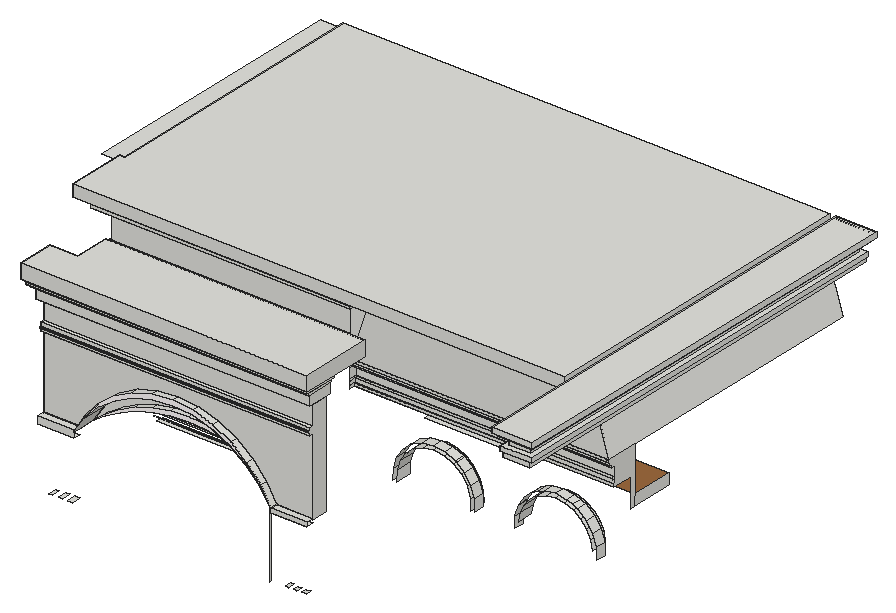
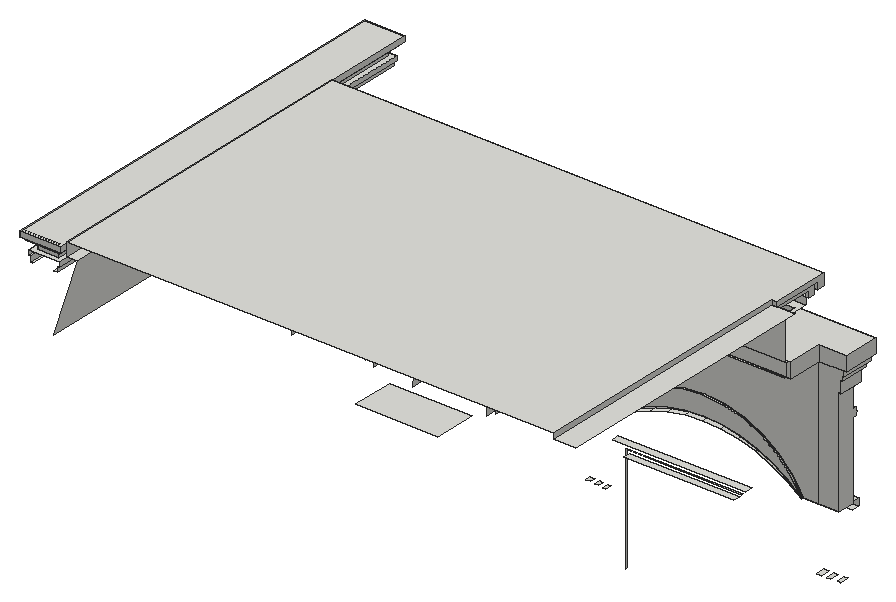
# SketchUp Ruby script. Lengths in millimetres.
U = 1.mm
M = Sketchup.active_model
def pt(a) = Geom::Point3d.new(a.map { |v| v * U })
def face(e, loops, mat)
  f = e.add_face(loops[0].map { |a| pt(a) })
  loops[1..].each { |l| e.add_face(l.map { |a| pt(a) }).erase! }
  f.material = f.back_material = mat if mat
  f
end
# faces: each face lists its corners as indices into pts; further lists are holes
def faces(e, pts, list, mat = nil) = list.each { |f| face(e, (f[0].is_a?(Array) ? f : [f]).map { |l| l.map { |i| pts[i] } }, mat) }
# xy, xz, yz: faces in a plane at the given z, y or x. An outline is a flat list of corners, or four numbers for a rectangle; further outlines are holes
def ring(l) = l.size == 4 ? [[l[0], l[1]], [l[2], l[1]], [l[2], l[3]], [l[0], l[3]]] : l.each_slice(2).to_a
def flat(e, list, mat, &to3) = list.each { |f| face(e, (f[0].is_a?(Array) ? f : [f]).map { |l| ring(l).map { |u, v| to3.(u, v) } }, mat) }
def xy(e, z, list, mat = nil) = flat(e, list, mat) { |x, y| [x, y, z] }
def xz(e, y, list, mat = nil) = flat(e, list, mat) { |x, z| [x, y, z] }
def yz(e, x, list, mat = nil) = flat(e, list, mat) { |y, z| [x, y, z] }
def lines(e, pts, list) = list.each { |a, b| e.add_line(pt(pts[a]), pt(pts[b])) }
# prism: a flat outline (further loops are holes) pulled along v
def prism(e, loops, v, mat = nil)
  f = face(e, loops, mat); d = Geom::Vector3d.new(v.map { |x| x * U })
  f.pushpull(f.normal.samedirection?(d) ? d.length : -d.length)
end
def box(e, o, s, mat = nil) = prism(e, [[o, [o[0] + s[0], o[1], o[2]], [o[0] + s[0], o[1] + s[1], o[2]], [o[0], o[1] + s[1], o[2]]]], [0, 0, s[2]], mat)
def at(x, y, z, deg = 0) = Geom::Transformation.translation(pt([x, y, z])) * Geom::Transformation.rotation(ORIGIN, Z_AXIS, deg.degrees)
def axes(o, x, y, z) = Geom::Transformation.new([*x, 0, *y, 0, *z, 0, *pt(o).to_a, 1])
def part(name) = M.definitions.add(name)
# library, detail: a bought-in or finely detailed component or shape, given as its bounding box
def library(name, o, s) = part(name).tap { |d| box(d.entities, o, s) }
def detail(e, o, s) = box(e.add_group.entities, o, s)
def put(e, d, t, mat = nil) = e.add_instance(d, t).tap { |i| i.material = mat if mat }
def group(e, t, mat = nil) = e.add_group.tap { |g| g.transformation = t; g.material = mat if mat }.entities
root = M.entities
M.materials.add("[0010_Snow]").color = [255, 250, 250]
M.materials.add("[Wood Floor]").color = [155, 105, 61]
xy(root,6858,[[4330.2,9852.4,4415.9,10085.7],[4585.1,9852.4,4702.2,10104.8],[4850.6,9852.4,4980.7,10104.8],[10956.8,9852.4,11053.6,10033.3]])
xy(root,6861.6,[[11185.3,9852.4,11289.9,10007.9]])
xy(root,6872.3,[[11425.8,9852.4,11548,9993.6]])
xy(root,8639.6,[[4179.9,9646,5191.1,9852.4]])
xy(root,8713.5,[[10715.6,9646,11726.9,9852.4]])
xy(root,8794.8,[[4179.9,9852.4,5191.1,10323.8],[10715.6,9852.4,11726.9,10323.8]])
xy(root,8794.9,[[6306,11161,9386.9,11364.2]])
xy(root,8828.1,[[10715.6,9646,11726.9,9852.4]])
xy(root,8850.3,[[4179.9,9646,5191.1,9852.4]])
xy(root,8890.1,[[6210.7,11161,9482.2,11195.9]])
xy(root,9007,[[6093.9,11161,9599.1,11195.9]])
xy(root,9121.9,[[5979,11161,9713.9,11364.2]])
xy(root,9853.1,[[11972,13477.1,14275.5,14659.8]])
xy(root,10869.6,[[11545.3,12281.7,18830,13477.1]],"[Wood Floor]")
xy(root,10955.7,[[4179.9,9739.6,11726.9,9852.4]])
xy(root,11034.9,[[4179.9,9709.5,11726.9,9739.6]])
xy(root,11068.4,[[4179.9,9709.5,11726.9,9739.6]])
xy(root,11161.7,[[4179.9,9739.6,11726.9,9852.4]])
xy(root,11371.3,[[11545.3,11530.8,18830,12124.7]])
xy(root,11443.4,[[11545.3,11530.8,18830,11557.8]])
xy(root,11540.8,[[11545.3,11557.8,18830,11575.3]])
xy(root,11603.9,[[11545.3,11575.3,18830,11588]])
xy(root,11778.1,[[4129.1,9644.4,11823.7,9852.4],[4129.1,9852.4,4179.9,10323.8],[11726.9,9852.4,11823.7,10323.8]])
xy(root,11896,[[11545.3,11461,18830,11588]])
xy(root,11974,[[11545.3,11403.8,18830,11461]])
xy(root,12064,[[11545.3,11361,18830,11403.8]])
xy(root,12112.6,[[4084.6,9523.7,11866.6,9644.4],[4084.6,9644.4,4129.1,10323.8],[11823.7,9644.4,11866.6,10323.8]])
xy(root,12141.6,[[11545.3,11361,18830,11364.2]])
xy(root,12233.2,[[4043.4,9387.2,4084.6,10323.8],[4084.6,9387.2,11928.5,9523.7],[11866.6,9523.7,11928.5,10323.8]])
xy(root,12370.5,[[3973.5,9282.4,4043.4,10323.8],[4043.4,9282.4,4129.1,9387.2],[4129.1,9282.4,12022.1,9387.2],[4043.4,9387.2,11928.5,10323.8],[11928.5,9387.2,12022.1,11300.2],
  [4747.3,10323.8,11928.5,11300.2],[4869.5,11300.2,11545.3,11364.2]])
xy(root,12768.3,[[4815.5,11300.2,4869.5,11364.2],[4869.5,11300.2,11545.3,11364.2]])
xy(root,12777.8,[[3973.5,9282.4,12022.1,9282.4,12022.1,11300.2,4747.3,11300.2,4747.3,10323.8,3973.5,10323.8]])
xy(root,13750.5,[[4994.2,10870.4,11774.4,11364.2]])
xy(root,13753.6,[[18742.6,7762.1,18830,19554.1],[18830,7762.1,19424.7,8551.1],[19424.7,7762.1,19486.6,19554.1]])
xy(root,13883.8,[[4869.5,10648.2,4869.5,11364.2,4994.2,11364.2,4994.2,10870.4,11774.4,10870.4,11774.4,11364.2,12134.1,11364.2,12134.1,10648.2]])
xy(root,13895.1,[[18683.9,7733.5,18742.6,19554.1],[18742.6,7733.5,19486.6,7762.1],[19486.6,7733.5,19558,19554.1]])
xy(root,14035.1,[[[18683.9,7733.5,19558,19554.1],[18824,7873.6,19417.9,19414]]])
xy(root,14097,[[4775.8,10468.8,12253.3,10648.2],[12134.1,10648.2,12206.1,11364.2]])
xy(root,14236.7,[[12253.3,10468.8,18173.1,11364.2],[18173.1,10468.8,18485.5,19554.1],[12206.1,10648.2,12253.3,11364.2]])
xy(root,14263.7,[[4671.1,10238.6,18485.5,10468.8]])
xy(root,14271.6,[[[18646.9,7696.6,19595,19591],[18824,7873.6,19417.9,19414]]])
xy(root,14284.3,[[4775.8,10648.2,4869.5,11889.6]])
xy(root,14362.1,[[[18558.1,7607.8,19683.8,19679.8],[18646.9,7696.6,19595,19591]]])
xy(root,14452.6,[[4671.1,10468.8,4775.8,11889.6],[4179.9,11889.6,4815.5,19554.1]])
xy(root,14509.8,[[18558.1,7607.8,19683.8,19679.8]])
xy(root,14595.5,[[4671.1,10238.6,18485.5,10238.6,18485.5,19554.1,4815.5,19554.1,4815.5,11889.6,4671.1,11889.6]])
xz(root,7607.8,[[18558.1,14362.1,19683.8,14509.8]])
xz(root,7696.6,[[18646.9,14271.6,19595,14362.1]])
xz(root,7733.5,[[18683.9,13895.1,19558,14035.1]])
xz(root,7762.1,[[18742.6,13753.6,19486.6,13895.1]])
xz(root,7873.6,[[18824,14035.1,19417.9,14271.6]])
xz(root,9282.4,[[3973.5,12370.5,12022.1,12777.8]])
xz(root,9387.2,[[4043.4,12233.2,11928.5,12370.5]])
xz(root,9523.7,[[4084.6,12112.6,11866.6,12233.2]])
xz(root,9644.4,[[4129.1,11778.1,11823.7,12112.6]])
xz(root,9646,[[4179.9,8639.6,5191.1,8850.3],[10715.6,8713.5,11726.9,8828.1]])
xz(root,9646,[[5191.1,8794.8,5502.6,9261.5,5892.1,9665.5,6347.2,9993.9,6853.3,10236.2,7394.5,10384.7,7953.4,10434.8,8512.3,10384.7,9053.4,10236.2,9559.6,9993.9,10014.6,9665.5,10404.1,9261.5,10715.6,8794.8,10427.2,9295,10049.2,9731.6,9595.4,10088.7,9082.2,10353.4,8528.2,10516.2,7953.4,10571.1,7378.5,10516.2,6824.5,10353.4,6311.3,10088.7,5857.5,9731.6,5479.6,9295]],"[0010_Snow]")
xz(root,9709.5,[[4179.9,11034.9,11726.9,11068.4]])
xz(root,9739.6,[[4179.9,10955.7,11726.9,11034.9],[4179.9,11068.4,11726.9,11161.7]])
xz(root,9852.4,[[4179.9,8794.8,5191.1,8850.3],[5191.1,8794.8,5479.6,9295,5857.5,9731.6,6311.3,10088.7,6824.5,10353.4,7378.5,10516.2,7953.4,10571.1,8528.2,10516.2,9082.2,10353.4,9595.4,10088.7,10049.2,9731.6,10427.2,9295,10715.6,8794.8,10715.6,8828.1,11726.9,8828.1,11726.9,10955.7,4179.9,10955.7,4179.9,8850.3,5191.1,8850.3],[10715.6,8794.8,11726.9,8828.1],[4179.9,11161.7,11726.9,11778.1]])
xz(root,10212.7,[[5191.1,8794.8,5579.2,9123.1,6006,9399.3,6464.4,9618.9,6947,9778.4,7446.1,9875.2,7953.4,9907.6,8460.7,9875.2,8959.7,9778.4,9442.4,9618.9,9900.8,9399.3,10327.5,9123.1,10715.6,8794.8,10312.3,9087.1,9878.4,9331.6,9419.5,9525.2,8941.5,9665.2,8450.7,9750,7953.4,9778.4,7456.1,9750,6965.3,9665.2,6487.3,9525.2,6028.4,9331.6,5594.4,9087.1]],"[0010_Snow]")
xz(root,10238.6,[[4671.1,14263.7,18485.5,14595.5]])
xz(root,10323.8,[[4179.9,8794.8,4179.9,11778.1,4129.1,11778.1,4129.1,12112.6,4084.6,12112.6,4084.6,12233.2,4043.4,12233.2,4043.4,12370.5,4747.3,12370.5,4747.3,8794.8],[4747.3,8794.8,4747.3,12370.5,11928.5,12370.5,11928.5,12233.2,11866.6,12233.2,11866.6,12112.6,11823.7,12112.6,11823.7,11778.1,11726.9,11778.1,11726.9,8794.8,10715.6,8794.8,10404.1,9261.5,10014.6,9665.5,9559.6,9993.9,9053.4,10236.2,8512.3,10384.7,7953.4,10434.8,7394.5,10384.7,6853.3,10236.2,6347.2,9993.9,5892.1,9665.5,5502.6,9261.5,5191.1,8794.8],[3973.5,12370.5,4747.3,12777.8]])
xz(root,10381,[[5191.1,8794.8,5502.6,9261.5,5892.1,9665.5,6347.2,9993.9,6853.3,10236.2,7394.5,10384.7,7953.4,10434.8,8512.3,10384.7,9053.4,10236.2,9559.6,9993.9,10014.6,9665.5,10404.1,9261.5,10715.6,8794.8,10327.5,9123.1,9900.8,9399.3,9442.4,9618.9,8959.7,9778.4,8460.7,9875.2,7953.4,9907.6,7446.1,9875.2,6947,9778.4,6464.4,9618.9,6006,9399.3,5579.2,9123.1]])
xz(root,10468.8,[[4775.8,14097,12253.3,14097,12253.3,14236.7,18485.5,14236.7,18485.5,14263.7,4775.8,14263.7],[4671.1,14263.7,4775.8,14452.6]])
xz(root,10648.2,[[4869.5,13883.8,12134.1,14097],[4775.8,14097,4869.5,14284.3],[12206.1,14097,12253.3,14236.7]])
xz(root,10870.4,[[4994.2,13750.5,11774.4,13883.8]])
xz(root,11300.2,[[4747.3,12370.5,4747.3,12777.8,4815.5,12777.8,4815.5,12768.3,4869.5,12768.3,4869.5,12370.5],[4869.5,12370.5,11545.3,12768.3],[11545.3,12370.5,12022.1,12777.8],[4815.5,12768.3,11545.3,12777.8]])
xz(root,11361,[[11545.3,12064,18830,12141.6]])
xz(root,11364.2,[[11545.3,12141.6,12134.1,13883.8,12206.1,14097,12253.3,14236.7,12206.1,14236.7,12206.1,14097,12134.1,14097,12134.1,13883.8,11774.4,13883.8,11774.4,13750.5,11545.3,13750.5],[11545.3,12141.6,18830,12141.6,18173.1,14236.7,12253.3,14236.7,12206.1,14097,12134.1,13883.8],[4869.5,12768.3,11545.3,12768.3,11545.3,13750.5,4994.2,13750.5,4994.2,13883.8,4869.5,13883.8]])
xz(root,11403.8,[[11545.3,11974,18830,12064]])
xz(root,11461,[[11545.3,11896,18830,11974]])
xz(root,11530.8,[[11545.3,11371.3,18830,11443.4]])
xz(root,11557.8,[[11545.3,11443.4,18830,11540.8]])
xz(root,11575.3,[[11545.3,11540.8,18830,11603.9]])
xz(root,11588,[[11545.3,11603.9,18830,11896]])
xz(root,11889.6,[[4671.1,14452.6,4815.5,14595.5]])
xz(root,19414,[[18824,14035.1,19417.9,14271.6],[18824,14271.6,19417.9,14362.1]])
xz(root,19591,[[18646.9,14271.6,19595,14362.1],[18646.9,14362.1,19595,14509.8]])
xz(root,19679.8,[[18558.1,14362.1,19683.8,14509.8]])
yz(root,3973.5,[[9282.4,12370.5,10323.8,12777.8]])
yz(root,4043.4,[[9387.2,12233.2,10323.8,12370.5]])
yz(root,4084.6,[[9523.7,12112.6,10323.8,12233.2]])
yz(root,4129.1,[[9644.4,11778.1,10323.8,12112.6]])
yz(root,4179.9,[[9852.4,8794.8,9852.4,10955.7,9739.6,10955.7,9739.6,11034.9,9709.5,11034.9,9709.5,11068.4,9739.6,11068.4,9739.6,11161.7,9852.4,11161.7,9852.4,11778.1,10323.8,11778.1,10323.8,8794.8]])
yz(root,4671.1,[[10238.6,14263.7,10238.6,14595.5,11889.6,14595.5,11889.6,14452.6,10468.8,14452.6,10468.8,14263.7]])
yz(root,4747.3,[[10323.8,12370.5,11300.2,12777.8]])
yz(root,4775.8,[[10468.8,14097,10468.8,14452.6,11889.6,14452.6,11889.6,14284.3,10648.2,14284.3,10648.2,14097]])
yz(root,4815.5,[[11889.6,14452.6,19554.1,14595.5]])
yz(root,4994.2,[[10870.4,13750.5,11364.2,13883.8]])
yz(root,5191.1,[[9646,8794.8,9852.4,8850.3]])
yz(root,9482.2,[[11161,5877.4,11195.9,8890.1]])
yz(root,10715.6,[[9646,8794.8,9852.4,8828.1]])
yz(root,11545.3,[[11364.2,11371.3,11530.8,11443.4],[11364.2,11443.4,11557.8,11540.8],[11364.2,11540.8,11575.3,11603.9],[11364.2,11603.9,11588,11896],[11364.2,11896,11461,11974],
  [11364.2,11974,11403.8,12064],[11361,12064,11364.2,12141.6],[11300.2,12370.5,11364.2,12768.3]])
yz(root,11726.9,[[9852.4,8794.8,10323.8,8794.8,10323.8,11778.1,9852.4,11778.1,9852.4,11161.7,9739.6,11161.7,9739.6,11068.4,9709.5,11068.4,9709.5,11034.9,9739.6,11034.9,9739.6,10955.7,9852.4,10955.7]])
yz(root,11774.4,[[10870.4,13750.5,11364.2,13883.8]])
yz(root,11823.7,[[9644.4,11778.1,10323.8,12112.6]])
yz(root,11866.6,[[9523.7,12112.6,10323.8,12233.2]])
yz(root,11928.5,[[9387.2,12233.2,10323.8,12370.5]])
yz(root,12022.1,[[9282.4,12370.5,11300.2,12777.8]])
yz(root,12134.1,[[10648.2,13883.8,11364.2,14097]])
yz(root,12206.1,[[10648.2,14097,11364.2,14236.7]])
yz(root,12253.3,[[10468.8,14097,10648.2,14236.7]])
yz(root,18485.5,[[10468.8,14236.7,19554.1,14236.7,19554.1,14595.5,10238.6,14595.5,10238.6,14263.7,10468.8,14263.7]])
yz(root,18558.1,[[7607.8,14362.1,19679.8,14509.8]])
yz(root,18646.9,[[7696.6,14271.6,19591,14362.1]])
yz(root,18683.9,[[7733.5,13895.1,19554.1,14035.1]])
yz(root,18742.6,[[7762.1,13753.6,19554.1,13895.1]])
yz(root,18824,[[7873.6,14035.1,19414,14271.6]])
yz(root,18830,[[12124.7,10572.8,12281.7,10572.8,12281.7,12141.6,11361,12141.6,11361,12064,11403.8,12064,11403.8,11974,11461,11974,11461,11896,11588,11896,11588,11603.9,11575.3,11603.9,11575.3,11540.8,11557.8,11540.8,11557.8,11443.4,11530.8,11443.4,11530.8,11371.3,12124.7,11371.3],[12281.7,10572.8,13477.1,10869.6]])
yz(root,19417.9,[[7873.6,14035.1,19414,14271.6]])
yz(root,19486.6,[[7762.1,13753.6,19554.1,13895.1]])
yz(root,19558,[[7733.5,13895.1,19554.1,14035.1]])
yz(root,19595,[[7696.6,14271.6,19591,14362.1]])
yz(root,19683.8,[[7607.8,14362.1,19679.8,14509.8]])
p = [[5502.6,10323.8,9261.5],[5502.6,9646,9261.5],[5191.1,9646,8794.8],[5191.1,9852.4,8794.8],[5191.1,10212.7,8794.8],[5191.1,10323.8,8794.8],
  [5479.6,9852.4,9295],[5479.6,9646,9295],[10404.1,10323.8,9261.5],[10715.6,10323.8,8794.8],[10715.6,10212.7,8794.8],[10715.6,9852.4,8794.8],
  [10715.6,9646,8794.8],[10404.1,9646,9261.5],[10427.2,9852.4,9295],[10427.2,9646,9295],[5594.4,10381,9087.1],[5191.1,10381,8794.8],
  [5594.4,10212.7,9087.1],[5579.2,10381,9123.1],[5579.2,10212.7,9123.1],[10715.6,10381,8794.8],[10312.3,10381,9087.1],[10312.3,10212.7,9087.1],
  [10327.5,10381,9123.1],[10327.5,10212.7,9123.1],[5502.6,10381,9261.5],[10404.1,10381,9261.5],[6028.4,10381,9331.6],[6028.4,10212.7,9331.6],
  [9878.4,10381,9331.6],[9878.4,10212.7,9331.6],[6006,10381,9399.3],[6006,10212.7,9399.3],[9900.8,10381,9399.3],[9900.8,10212.7,9399.3],
  [15814.7,12124.7,9462],[15805,12124.7,9139.4],[15805,11848.5,9139.4],[15814.7,11848.5,9462],[18102.6,12124.7,9139.4],[18092.9,12124.7,9462],
  [18092.9,11848.5,9462],[18102.6,11848.5,9139.4],[12506.8,12281.7,9453.2],[12506.8,11848.5,9453.2],[12495.4,11848.5,9150.1],[12495.4,12281.7,9150.1],
  [14574.9,12281.7,9150.1],[14574.9,11848.5,9150.1],[14563.5,11848.5,9453.2],[14563.5,12281.7,9453.2],[12400.2,12124.7,9472.3],[12388.2,12124.7,9152.2],
  [12388.2,11848.5,9152.2],[12400.2,11848.5,9472.3],[14682.1,12124.7,9152.2],[14670.1,12124.7,9472.3],[14670.1,11848.5,9472.3],[14682.1,11848.5,9152.2],
  [5892.1,10323.8,9665.5],[5892.1,9646,9665.5],[10014.6,9646,9665.5],[10014.6,10323.8,9665.5],[5892.1,10381,9665.5],[10014.6,10381,9665.5],
  [5857.5,9852.4,9731.6],[5857.5,9646,9731.6],[10049.2,9852.4,9731.6],[10049.2,9646,9731.6],[6487.3,10381,9525.2],[6487.3,10212.7,9525.2],
  [9419.5,10381,9525.2],[9419.5,10212.7,9525.2],[15968.2,12281.7,9601.1],[15968.2,11848.5,9601.1],[15917.1,11848.5,9347.6],[15917.1,12281.7,9347.6],
  [17990.5,12281.7,9347.6],[17990.5,11848.5,9347.6],[17939.4,11848.5,9601.1],[17939.4,12281.7,9601.1],[6464.4,10381,9618.9],[6464.4,10212.7,9618.9],
  [9442.4,10381,9618.9],[9442.4,10212.7,9618.9],[12597.2,12281.7,9729],[12597.2,11848.5,9729],[14473.2,11848.5,9729],[14473.2,12281.7,9729],
  [15913.2,12124.7,9769.3],[15913.2,11848.5,9769.3],[17994.4,12124.7,9769.3],[17994.4,11848.5,9769.3],[12499.9,12124.7,9776.7],[12499.9,11848.5,9776.7],
  [14570.4,12124.7,9776.7],[14570.4,11848.5,9776.7],[6965.3,10381,9665.2],[6965.3,10212.7,9665.2],[8941.5,10381,9665.2],[8941.5,10212.7,9665.2],
  [16080.3,12281.7,9834.2],[16080.3,11848.5,9834.2],[17827.3,11848.5,9834.2],[17827.3,12281.7,9834.2],[6947,10381,9778.4],[6947,10212.7,9778.4],
  [8959.7,10381,9778.4],[8959.7,10212.7,9778.4],[7456.1,10381,9750],[7456.1,10212.7,9750],[8450.7,10381,9750],[8450.7,10212.7,9750],
  [6347.2,10323.8,9993.9],[6347.2,9646,9993.9],[9559.6,9646,9993.9],[9559.6,10323.8,9993.9],[6347.2,10381,9993.9],[9559.6,10381,9993.9],
  [12759.9,12281.7,9969.4],[12759.9,11848.5,9969.4],[14310.4,11848.5,9969.4],[14310.4,12281.7,9969.4],[6311.3,9852.4,10088.7],[6311.3,9646,10088.7],
  [9595.4,9852.4,10088.7],[9595.4,9646,10088.7],[7953.4,10381,9778.4],[7953.4,10212.7,9778.4],[15917.1,12124.7,9775.1],[15917.1,11848.5,9775.1],
  [17990.5,12124.7,9775.1],[17990.5,11848.5,9775.1],[16092.8,12124.7,10037.4],[16092.8,11848.5,10037.4],[17814.8,12124.7,10037.4],[17814.8,11848.5,10037.4],
  [12679.5,12124.7,10042],[12679.5,11848.5,10042],[14390.8,12124.7,10042],[14390.8,11848.5,10042],[7446.1,10381,9875.2],[7446.1,10212.7,9875.2],
  [8460.7,10381,9875.2],[8460.7,10212.7,9875.2],[16246.5,12281.7,10032.4],[16246.5,11848.5,10032.4],[17661.1,11848.5,10032.4],[17661.1,12281.7,10032.4],
  [7953.4,10381,9907.6],[7953.4,10212.7,9907.6],[12976,12281.7,10150.3],[12976,11848.5,10150.3],[14094.3,11848.5,10150.3],[14094.3,12281.7,10150.3],
  [6853.3,10323.8,10236.2],[6853.3,9646,10236.2],[9053.4,9646,10236.2],[9053.4,10323.8,10236.2],[6853.3,10381,10236.2],[9053.4,10381,10236.2],
  [16456.4,12281.7,10183.4],[16456.4,11848.5,10183.4],[17451.2,11848.5,10183.4],[17451.2,12281.7,10183.4],[16339.6,12124.7,10245.4],[16339.6,11848.5,10245.4],
  [17568,12124.7,10245.4],[17568,11848.5,10245.4],[12907.2,12124.7,10232.5],[12907.2,11848.5,10232.5],[14163.1,12124.7,10232.5],[14163.1,11848.5,10232.5],
  [6824.5,9852.4,10353.4],[6824.5,9646,10353.4],[9082.2,9852.4,10353.4],[9082.2,9646,10353.4],[12982.5,12281.7,10155.7],[12982.5,11848.5,10155.7],
  [14087.8,11848.5,10155.7],[14087.8,12281.7,10155.7],[13247.7,12281.7,10273.5],[13247.7,11848.5,10273.5],[13822.6,11848.5,10273.5],[13822.6,12281.7,10273.5],
  [16697.2,12281.7,10277.9],[16697.2,11848.5,10277.9],[17210.4,11848.5,10277.9],[17210.4,12281.7,10277.9],[12925.2,12124.7,10247.6],[12925.2,11848.5,10247.6],
  [14145.1,12124.7,10247.6],[14145.1,11848.5,10247.6],[7394.5,10323.8,10384.7],[7394.5,9646,10384.7],[8512.3,9646,10384.7],[8512.3,10323.8,10384.7],
  [7394.5,10381,10384.7],[8512.3,10381,10384.7],[16484.3,12124.7,10310.1],[16484.3,11848.5,10310.1],[17423.3,12124.7,10310.1],[17423.3,11848.5,10310.1],
  [13217.9,12124.7,10377.7],[13217.9,11848.5,10377.7],[13852.4,12124.7,10377.7],[13852.4,11848.5,10377.7],[13535.2,12281.7,10313.9],[13535.2,11848.5,10313.9],
  [16953.8,12281.7,10310.1],[16953.8,11848.5,10310.1],[16634.2,12124.7,10377.1],[16634.2,11848.5,10377.1],[17273.4,12124.7,10377.1],[17273.4,11848.5,10377.1],
  [7378.5,9852.4,10516.2],[7378.5,9646,10516.2],[8528.2,9852.4,10516.2],[8528.2,9646,10516.2],[16953.8,12124.7,10422.2],[16953.8,11848.5,10422.2],
  [13535.2,12124.7,10422.2],[13535.2,11848.5,10422.2],[7953.4,10323.8,10434.8],[7953.4,9646,10434.8],[7953.4,10381,10434.8],[7953.4,9852.4,10571.1],
  [7953.4,9646,10571.1],[18173.1,11364.2,14236.7],[18830,11364.2,12141.6],[18830,12281.7,12141.6],[18830,19554.1,12141.6],[18173.1,19554.1,14236.7],
  [4179.9,9852.4,6858],[4117.8,9852.4,6858],[11545.3,12281.7,10869.6],[11545.3,12281.7,11166.5],[19417.9,7873.6,14271.6],[19417.9,7873.6,14362.1],
  [18824,7873.6,14271.6],[18824,7873.6,14362.1],[18646.9,7696.6,14362.1],[18646.9,7696.6,14509.8],[19595,7696.6,14362.1],[19595,7696.6,14509.8]]
faces(root,p,[[0,1,2,3,4,5],[6,3,2,7],[8,9,10,11,12,13],[11,14,15,12],[16,17,5,4,18],[17,19,20,4,5],[21,22,23,10,9],[24,21,9,10,25],
  [5,0,26,17],[8,9,21,27],[28,16,18,29],[22,30,31,23],[19,32,33,20],[34,24,25,35],[36,37,38,39],[40,41,42,43],
  [44,45,46,47],[48,49,50,51],[52,53,54,55],[56,57,58,59],[60,61,1,0],[8,13,62,63],[0,60,64,26],[63,8,27,65],
  [66,6,7,67],[14,68,69,15],[70,28,29,71],[30,72,73,31],[74,75,76,77],[78,79,80,81],[32,82,83,33],[84,34,35,85],
  [86,87,45,44],[51,50,88,89],[90,36,39,91],[41,92,93,42],[94,52,55,95],[57,96,97,58],[98,70,71,99],[72,100,101,73],
  [102,103,75,74],[81,80,104,105],[82,106,107,83],[108,84,85,109],[110,98,99,111],[100,112,113,101],[114,115,61,60],[63,62,116,117],
  [60,114,118,64],[117,63,65,119],[120,121,87,86],[89,88,122,123],[124,66,67,125],[68,126,127,69],[128,110,111,129],[112,128,129,113],
  [130,90,91,131],[92,132,133,93],[134,130,131,135],[132,136,137,133],[138,94,95,139],[96,140,141,97],[106,142,143,107],[144,108,109,145],
  [146,147,103,102],[105,104,148,149],[142,150,151,143],[150,144,145,151],[152,153,121,120],[123,122,154,155],[156,157,115,114],[117,116,158,159],
  [114,156,160,118],[159,117,119,161],[162,163,147,146],[149,148,164,165],[166,134,135,167],[136,168,169,137],[170,138,139,171],[140,172,173,141],
  [174,124,125,175],[126,176,177,127],[178,179,153,152],[155,154,180,181],[182,183,179,178],[181,180,184,185],[186,187,163,162],[165,164,188,189],
  [190,170,171,191],[172,192,193,173],[194,195,157,156],[159,158,196,197],[156,194,198,160],[197,159,161,199],[200,166,167,201],[168,202,203,169],
  [204,190,191,205],[192,206,207,193],[208,209,183,182],[185,184,209,208],[210,211,187,186],[189,188,211,210],[212,200,201,213],[202,214,215,203],
  [216,174,175,217],[176,218,219,177],[220,212,213,221],[214,220,221,215],[222,204,205,223],[206,222,223,207],[224,225,195,194],[197,196,225,224],
  [194,224,226,198],[224,197,199,226],[227,216,217,228],[218,227,228,219],[229,230,231,232,233]])
lines(root,p,[[234,235],[236,237],[238,239],[240,241],[242,243],[244,245]])
